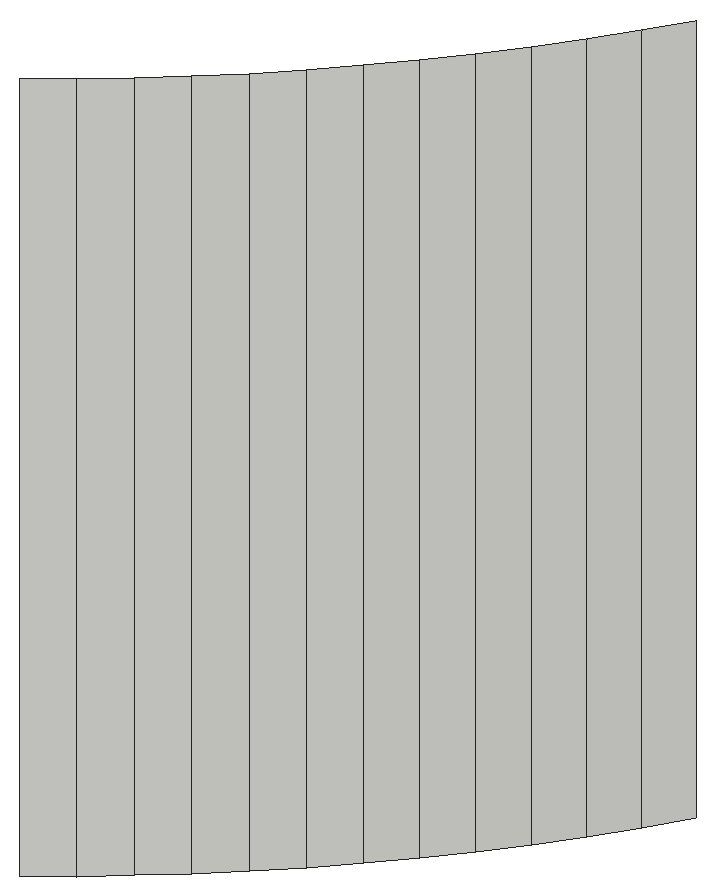
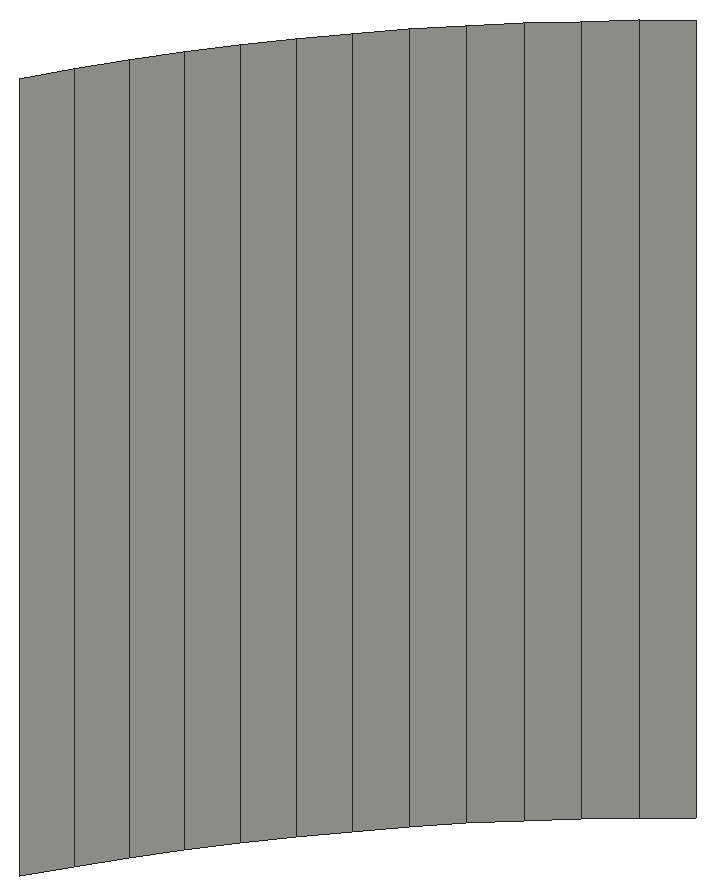
# SketchUp Ruby script. Lengths in inches.
U = 1.inch
M = Sketchup.active_model
def pt(a) = Geom::Point3d.new(a.map { |v| v * U })
def face(e, loops, mat)
  f = e.add_face(loops[0].map { |a| pt(a) })
  loops[1..].each { |l| e.add_face(l.map { |a| pt(a) }).erase! }
  f.material = f.back_material = mat if mat
  f
end
# faces: each face lists its corners as indices into pts; further lists are holes
def faces(e, pts, list, mat = nil) = list.each { |f| face(e, (f[0].is_a?(Array) ? f : [f]).map { |l| l.map { |i| pts[i] } }, mat) }
# xy, xz, yz: faces in a plane at the given z, y or x. An outline is a flat list of corners, or four numbers for a rectangle; further outlines are holes
def ring(l) = l.size == 4 ? [[l[0], l[1]], [l[2], l[1]], [l[2], l[3]], [l[0], l[3]]] : l.each_slice(2).to_a
def flat(e, list, mat, &to3) = list.each { |f| face(e, (f[0].is_a?(Array) ? f : [f]).map { |l| ring(l).map { |u, v| to3.(u, v) } }, mat) }
def xy(e, z, list, mat = nil) = flat(e, list, mat) { |x, y| [x, y, z] }
def xz(e, y, list, mat = nil) = flat(e, list, mat) { |x, z| [x, y, z] }
def yz(e, x, list, mat = nil) = flat(e, list, mat) { |y, z| [x, y, z] }
def lines(e, pts, list) = list.each { |a, b| e.add_line(pt(pts[a]), pt(pts[b])) }
# prism: a flat outline (further loops are holes) pulled along v
def prism(e, loops, v, mat = nil)
  f = face(e, loops, mat); d = Geom::Vector3d.new(v.map { |x| x * U })
  f.pushpull(f.normal.samedirection?(d) ? d.length : -d.length)
end
def box(e, o, s, mat = nil) = prism(e, [[o, [o[0] + s[0], o[1], o[2]], [o[0] + s[0], o[1] + s[1], o[2]], [o[0], o[1] + s[1], o[2]]]], [0, 0, s[2]], mat)
def at(x, y, z, deg = 0) = Geom::Transformation.translation(pt([x, y, z])) * Geom::Transformation.rotation(ORIGIN, Z_AXIS, deg.degrees)
def axes(o, x, y, z) = Geom::Transformation.new([*x, 0, *y, 0, *z, 0, *pt(o).to_a, 1])
def part(name) = M.definitions.add(name)
# library, detail: a bought-in or finely detailed component or shape, given as its bounding box
def library(name, o, s) = part(name).tap { |d| box(d.entities, o, s) }
def detail(e, o, s) = box(e.add_group.entities, o, s)
def put(e, d, t, mat = nil) = e.add_instance(d, t).tap { |i| i.material = mat if mat }
def group(e, t, mat = nil) = e.add_group.tap { |g| g.transformation = t; g.material = mat if mat }.entities
root = M.entities
p = [[152.03,231.78,357],[152.47,232.13,357],[152.47,232.13,348],[152.03,231.78,348],[152.9,232.5,357],[152.9,232.5,348],
  [153.32,232.88,357],[153.32,232.88,348],[153.73,233.27,357],[153.73,233.27,348],[154.12,233.68,357],[154.12,233.68,348],
  [154.5,234.1,357],[154.5,234.1,348],[154.87,234.53,357],[154.87,234.53,348],[155.22,234.97,357],[155.22,234.97,348],
  [155.5625,235.42,357],[155.5625,235.42,348],[155.89,235.88,357],[155.89,235.88,348],[156.2,236.36,357],[156.2,236.36,348],
  [156.49,236.84,357],[156.49,236.84,348]]
faces(root,p,[[0,1,2,3],[1,4,5,2],[4,6,7,5],[6,8,9,7],[8,10,11,9],[10,12,13,11],[12,14,15,13],[14,16,17,15],
  [16,18,19,17],[18,20,21,19],[20,22,23,21],[22,24,25,23]])
